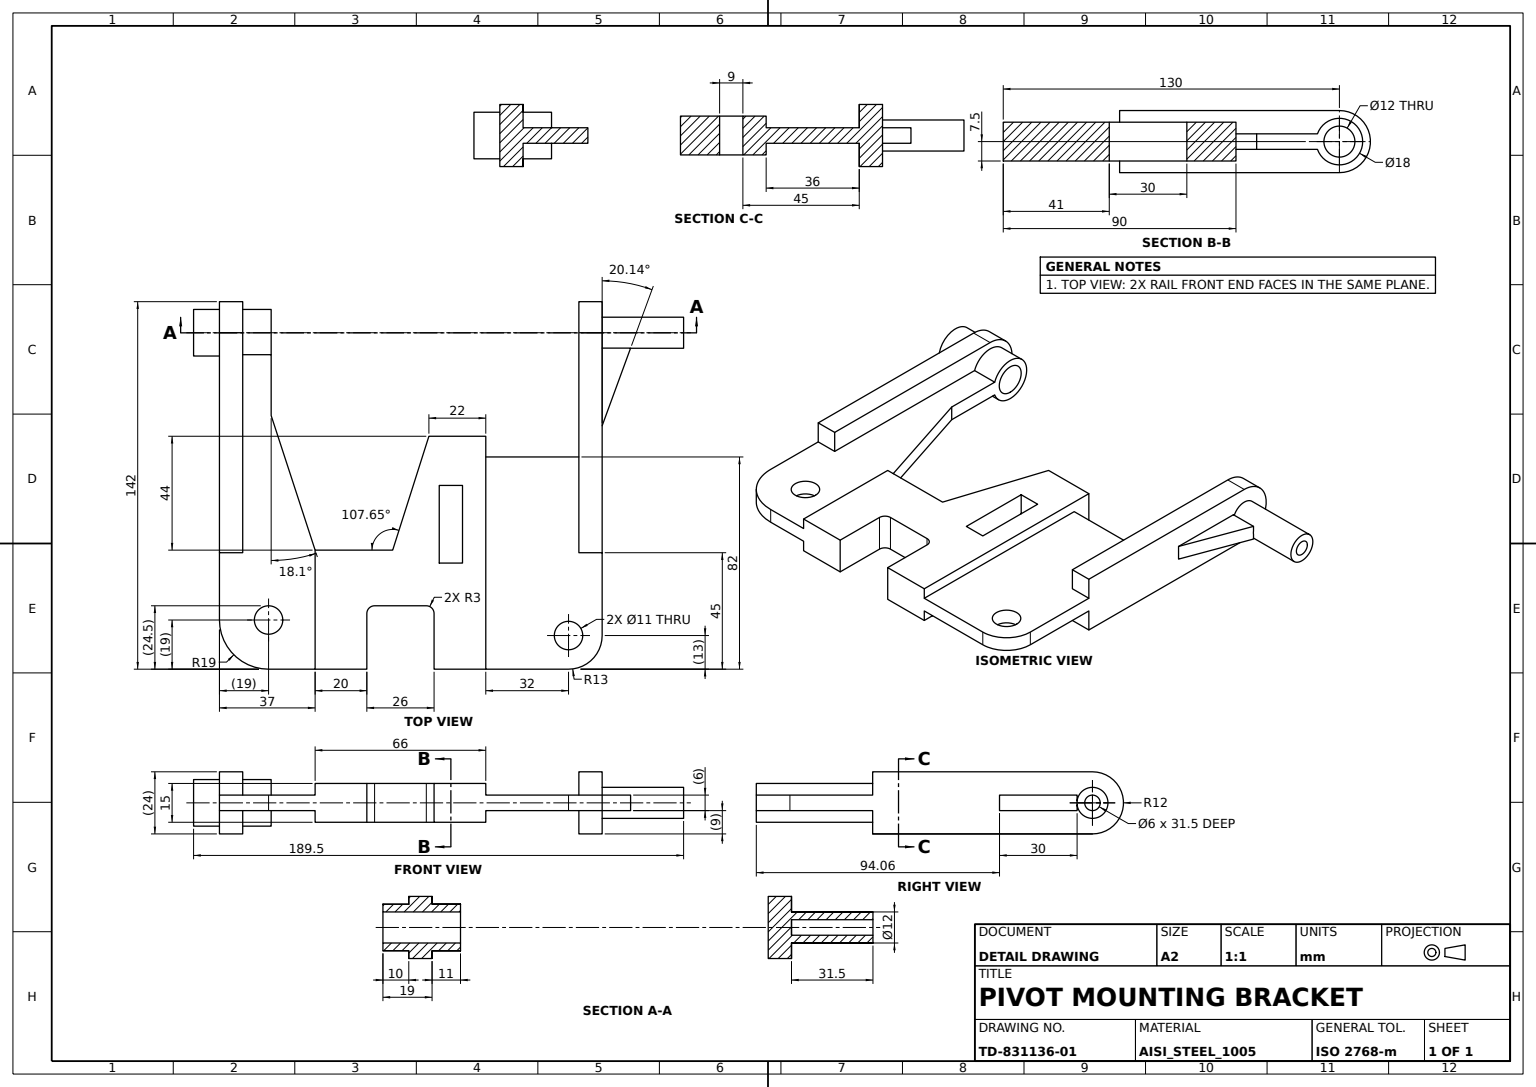
ISO-10303-21;
HEADER;
FILE_DESCRIPTION((''),'2;1');
FILE_NAME('','',(''),(''),'','','');
FILE_SCHEMA(('AUTOMOTIVE_DESIGN'));
ENDSEC;
DATA;
#1=APPLICATION_CONTEXT('');
#2=PRODUCT_CONTEXT('',#1,'mechanical');
#3=PRODUCT('','','',(#2));
#4=PRODUCT_DEFINITION_FORMATION('','',#3);
#5=PRODUCT_DEFINITION_CONTEXT('',#1,'design');
#6=PRODUCT_DEFINITION('','',#4,#5);
#7=PRODUCT_DEFINITION_SHAPE('','',#6);
#8=(LENGTH_UNIT()NAMED_UNIT(*)SI_UNIT(.MILLI.,.METRE.));
#9=(NAMED_UNIT(*)PLANE_ANGLE_UNIT()SI_UNIT($,.RADIAN.));
#10=(NAMED_UNIT(*)SI_UNIT($,.STERADIAN.)SOLID_ANGLE_UNIT());
#11=UNCERTAINTY_MEASURE_WITH_UNIT(LENGTH_MEASURE(0.005),#8,'distance_accuracy_value','');
#12=(GEOMETRIC_REPRESENTATION_CONTEXT(3)GLOBAL_UNCERTAINTY_ASSIGNED_CONTEXT((#11))GLOBAL_UNIT_ASSIGNED_CONTEXT((#8,#9,#10))REPRESENTATION_CONTEXT('',''));
#13=CARTESIAN_POINT('',(-80.,121.,0.));
#14=VERTEX_POINT('',#13);
#15=CARTESIAN_POINT('',(-80.,130.,0.));
#16=DIRECTION('',(-1.,0.,0.));
#17=DIRECTION('',(0.,-1.,0.));
#18=AXIS2_PLACEMENT_3D('',#15,#16,#17);
#19=CIRCLE('',#18,9.);
#20=EDGE_CURVE('',#14,#14,#19,.T.);
#21=ORIENTED_EDGE('',*,*,#20,.T.);
#22=EDGE_LOOP('',(#21));
#23=FACE_BOUND('',#22,.T.);
#24=CARTESIAN_POINT('',(-80.,130.,6.));
#25=VERTEX_POINT('',#24);
#26=DIRECTION('',(0.,0.,1.));
#27=AXIS2_PLACEMENT_3D('',#15,#16,#26);
#28=CIRCLE('',#27,6.);
#29=EDGE_CURVE('',#25,#25,#28,.F.);
#30=ORIENTED_EDGE('',*,*,#29,.T.);
#31=EDGE_LOOP('',(#30));
#32=FACE_BOUND('',#31,.T.);
#33=PLANE('',#27);
#34=ADVANCED_FACE('',(#23,#32),#33,.T.);
#35=CARTESIAN_POINT('',(78.,124.056727,-0.823106));
#36=VERTEX_POINT('',#35);
#37=CARTESIAN_POINT('',(89.,124.056727,-0.823106));
#38=VERTEX_POINT('',#37);
#39=CARTESIAN_POINT('',(109.5,124.056727,-0.823106));
#40=VECTOR('',#16,1000.);
#41=LINE('',#39,#40);
#42=EDGE_CURVE('',#36,#38,#41,.F.);
#43=ORIENTED_EDGE('',*,*,#42,.T.);
#44=CARTESIAN_POINT('',(89.,124.056727,-3.));
#45=VERTEX_POINT('',#44);
#46=CARTESIAN_POINT('',(89.,124.056727,3.));
#47=DIRECTION('',(0.,0.,-1.));
#48=VECTOR('',#47,1000.);
#49=LINE('',#46,#48);
#50=EDGE_CURVE('',#38,#45,#49,.T.);
#51=ORIENTED_EDGE('',*,*,#50,.T.);
#52=CARTESIAN_POINT('',(78.,124.056727,-3.));
#53=VERTEX_POINT('',#52);
#54=LINE('',#44,#40);
#55=EDGE_CURVE('',#45,#53,#54,.T.);
#56=ORIENTED_EDGE('',*,*,#55,.T.);
#57=CARTESIAN_POINT('',(78.,124.056727,3.));
#58=LINE('',#57,#48);
#59=EDGE_CURVE('',#36,#53,#58,.T.);
#60=ORIENTED_EDGE('',*,*,#59,.F.);
#61=EDGE_LOOP('',(#43,#51,#56,#60));
#62=FACE_BOUND('',#61,.T.);
#63=AXIS2_PLACEMENT_3D('',#46,#17,#47);
#64=PLANE('',#63);
#65=ADVANCED_FACE('',(#62),#64,.F.);
#66=CARTESIAN_POINT('',(-13.,21.5,-7.5));
#67=VERTEX_POINT('',#66);
#68=CARTESIAN_POINT('',(-13.,0.,-7.5));
#69=VERTEX_POINT('',#68);
#70=VECTOR('',#17,1000.);
#71=LINE('',#66,#70);
#72=EDGE_CURVE('',#67,#69,#71,.T.);
#73=ORIENTED_EDGE('',*,*,#72,.F.);
#74=CARTESIAN_POINT('',(-13.,21.5,7.5));
#75=VERTEX_POINT('',#74);
#76=LINE('',#74,#48);
#77=EDGE_CURVE('',#75,#67,#76,.T.);
#78=ORIENTED_EDGE('',*,*,#77,.F.);
#79=CARTESIAN_POINT('',(-13.,0.,7.5));
#80=VERTEX_POINT('',#79);
#81=LINE('',#74,#70);
#82=EDGE_CURVE('',#75,#80,#81,.T.);
#83=ORIENTED_EDGE('',*,*,#82,.T.);
#84=LINE('',#79,#48);
#85=EDGE_CURVE('',#80,#69,#84,.T.);
#86=ORIENTED_EDGE('',*,*,#85,.T.);
#87=EDGE_LOOP('',(#73,#78,#83,#86));
#88=FACE_BOUND('',#87,.T.);
#89=DIRECTION('',(1.,0.,0.));
#90=DIRECTION('',(0.,1.,0.));
#91=AXIS2_PLACEMENT_3D('',#74,#89,#90);
#92=PLANE('',#91);
#93=ADVANCED_FACE('',(#88),#92,.T.);
#94=CARTESIAN_POINT('',(-50.,98.,3.));
#95=VERTEX_POINT('',#94);
#96=CARTESIAN_POINT('',(-50.,98.,-3.));
#97=VERTEX_POINT('',#96);
#98=LINE('',#94,#48);
#99=EDGE_CURVE('',#95,#97,#98,.T.);
#100=ORIENTED_EDGE('',*,*,#99,.F.);
#101=CARTESIAN_POINT('',(-33.,46.,3.));
#102=VERTEX_POINT('',#101);
#103=DIRECTION('',(0.310738856,-0.950495325,0.));
#104=VECTOR('',#103,1000.);
#105=LINE('',#94,#104);
#106=EDGE_CURVE('',#95,#102,#105,.T.);
#107=ORIENTED_EDGE('',*,*,#106,.T.);
#108=CARTESIAN_POINT('',(-33.,46.,-3.));
#109=VERTEX_POINT('',#108);
#110=LINE('',#101,#48);
#111=EDGE_CURVE('',#102,#109,#110,.T.);
#112=ORIENTED_EDGE('',*,*,#111,.T.);
#113=LINE('',#96,#104);
#114=EDGE_CURVE('',#97,#109,#113,.T.);
#115=ORIENTED_EDGE('',*,*,#114,.F.);
#116=EDGE_LOOP('',(#100,#107,#112,#115));
#117=FACE_BOUND('',#116,.T.);
#118=DIRECTION('',(0.950495325,0.310738856,0.));
#119=DIRECTION('',(-0.310738856,0.950495325,0.));
#120=AXIS2_PLACEMENT_3D('',#94,#118,#119);
#121=PLANE('',#120);
#122=ADVANCED_FACE('',(#117),#121,.T.);
#123=CARTESIAN_POINT('',(69.,45.,-12.));
#124=VERTEX_POINT('',#123);
#125=CARTESIAN_POINT('',(69.,130.,-12.));
#126=VERTEX_POINT('',#125);
#127=VECTOR('',#90,1000.);
#128=LINE('',#123,#127);
#129=EDGE_CURVE('',#124,#126,#128,.T.);
#130=ORIENTED_EDGE('',*,*,#129,.T.);
#131=CARTESIAN_POINT('',(78.,130.,-12.));
#132=VERTEX_POINT('',#131);
#133=LINE('',#131,#40);
#134=EDGE_CURVE('',#132,#126,#133,.T.);
#135=ORIENTED_EDGE('',*,*,#134,.F.);
#136=CARTESIAN_POINT('',(78.,45.,-12.));
#137=VERTEX_POINT('',#136);
#138=LINE('',#136,#127);
#139=EDGE_CURVE('',#137,#132,#138,.T.);
#140=ORIENTED_EDGE('',*,*,#139,.F.);
#141=LINE('',#136,#40);
#142=EDGE_CURVE('',#137,#124,#141,.T.);
#143=ORIENTED_EDGE('',*,*,#142,.T.);
#144=EDGE_LOOP('',(#130,#135,#140,#143));
#145=FACE_BOUND('',#144,.T.);
#146=AXIS2_PLACEMENT_3D('',#136,#26,#17);
#147=PLANE('',#146);
#148=ADVANCED_FACE('',(#145),#147,.F.);
#149=CARTESIAN_POINT('',(-33.,0.,3.));
#150=VERTEX_POINT('',#149);
#151=CARTESIAN_POINT('',(-51.,0.,3.));
#152=VERTEX_POINT('',#151);
#153=LINE('',#149,#40);
#154=EDGE_CURVE('',#150,#152,#153,.T.);
#155=ORIENTED_EDGE('',*,*,#154,.T.);
#156=CARTESIAN_POINT('',(-51.,0.,-3.));
#157=VERTEX_POINT('',#156);
#158=LINE('',#151,#48);
#159=EDGE_CURVE('',#152,#157,#158,.T.);
#160=ORIENTED_EDGE('',*,*,#159,.T.);
#161=CARTESIAN_POINT('',(-33.,0.,-3.));
#162=VERTEX_POINT('',#161);
#163=LINE('',#161,#40);
#164=EDGE_CURVE('',#162,#157,#163,.T.);
#165=ORIENTED_EDGE('',*,*,#164,.F.);
#166=CARTESIAN_POINT('',(-33.,0.,-7.5));
#167=VERTEX_POINT('',#166);
#168=CARTESIAN_POINT('',(-33.,0.,7.5));
#169=LINE('',#168,#48);
#170=EDGE_CURVE('',#162,#167,#169,.T.);
#171=ORIENTED_EDGE('',*,*,#170,.T.);
#172=LINE('',#68,#40);
#173=EDGE_CURVE('',#69,#167,#172,.T.);
#174=ORIENTED_EDGE('',*,*,#173,.F.);
#175=ORIENTED_EDGE('',*,*,#85,.F.);
#176=VERTEX_POINT('',#168);
#177=LINE('',#79,#40);
#178=EDGE_CURVE('',#80,#176,#177,.T.);
#179=ORIENTED_EDGE('',*,*,#178,.T.);
#180=EDGE_CURVE('',#176,#150,#169,.T.);
#181=ORIENTED_EDGE('',*,*,#180,.T.);
#182=EDGE_LOOP('',(#155,#160,#165,#171,#174,#175,#179,#181));
#183=FACE_BOUND('',#182,.T.);
#184=AXIS2_PLACEMENT_3D('',#79,#17,#89);
#185=PLANE('',#184);
#186=ADVANCED_FACE('',(#183),#185,.T.);
#187=CARTESIAN_POINT('',(33.,0.,7.5));
#188=VERTEX_POINT('',#187);
#189=CARTESIAN_POINT('',(33.,0.,3.));
#190=VERTEX_POINT('',#189);
#191=LINE('',#187,#48);
#192=EDGE_CURVE('',#188,#190,#191,.T.);
#193=ORIENTED_EDGE('',*,*,#192,.F.);
#194=CARTESIAN_POINT('',(13.,0.,7.5));
#195=VERTEX_POINT('',#194);
#196=LINE('',#187,#40);
#197=EDGE_CURVE('',#188,#195,#196,.T.);
#198=ORIENTED_EDGE('',*,*,#197,.T.);
#199=CARTESIAN_POINT('',(13.,0.,-7.5));
#200=VERTEX_POINT('',#199);
#201=LINE('',#194,#48);
#202=EDGE_CURVE('',#195,#200,#201,.T.);
#203=ORIENTED_EDGE('',*,*,#202,.T.);
#204=CARTESIAN_POINT('',(33.,0.,-7.5));
#205=VERTEX_POINT('',#204);
#206=LINE('',#204,#40);
#207=EDGE_CURVE('',#205,#200,#206,.T.);
#208=ORIENTED_EDGE('',*,*,#207,.F.);
#209=CARTESIAN_POINT('',(33.,0.,-3.));
#210=VERTEX_POINT('',#209);
#211=EDGE_CURVE('',#210,#205,#191,.T.);
#212=ORIENTED_EDGE('',*,*,#211,.F.);
#213=CARTESIAN_POINT('',(65.,0.,-3.));
#214=VERTEX_POINT('',#213);
#215=LINE('',#213,#40);
#216=EDGE_CURVE('',#214,#210,#215,.T.);
#217=ORIENTED_EDGE('',*,*,#216,.F.);
#218=CARTESIAN_POINT('',(65.,0.,3.));
#219=VERTEX_POINT('',#218);
#220=LINE('',#218,#48);
#221=EDGE_CURVE('',#219,#214,#220,.T.);
#222=ORIENTED_EDGE('',*,*,#221,.F.);
#223=LINE('',#218,#40);
#224=EDGE_CURVE('',#219,#190,#223,.T.);
#225=ORIENTED_EDGE('',*,*,#224,.T.);
#226=EDGE_LOOP('',(#193,#198,#203,#208,#212,#217,#222,#225));
#227=FACE_BOUND('',#226,.T.);
#228=AXIS2_PLACEMENT_3D('',#187,#17,#89);
#229=PLANE('',#228);
#230=ADVANCED_FACE('',(#227),#229,.T.);
#231=CARTESIAN_POINT('',(78.,94.056727,3.));
#232=VERTEX_POINT('',#231);
#233=VERTEX_POINT('',#46);
#234=DIRECTION('',(0.344254649,0.938876316,0.));
#235=VECTOR('',#234,1000.);
#236=LINE('',#231,#235);
#237=EDGE_CURVE('',#232,#233,#236,.T.);
#238=ORIENTED_EDGE('',*,*,#237,.T.);
#239=VERTEX_POINT('',#57);
#240=LINE('',#46,#40);
#241=EDGE_CURVE('',#233,#239,#240,.T.);
#242=ORIENTED_EDGE('',*,*,#241,.T.);
#243=LINE('',#57,#70);
#244=EDGE_CURVE('',#239,#232,#243,.T.);
#245=ORIENTED_EDGE('',*,*,#244,.T.);
#246=EDGE_LOOP('',(#238,#242,#245));
#247=FACE_BOUND('',#246,.T.);
#248=CARTESIAN_POINT('',(0.,0.,3.));
#249=AXIS2_PLACEMENT_3D('',#248,#47,#16);
#250=PLANE('',#249);
#251=ADVANCED_FACE('',(#247),#250,.F.);
#252=CARTESIAN_POINT('',(69.,45.,-3.));
#253=VERTEX_POINT('',#252);
#254=CARTESIAN_POINT('',(69.,45.,12.));
#255=LINE('',#254,#48);
#256=EDGE_CURVE('',#253,#124,#255,.T.);
#257=ORIENTED_EDGE('',*,*,#256,.T.);
#258=ORIENTED_EDGE('',*,*,#142,.F.);
#259=CARTESIAN_POINT('',(78.,45.,-3.));
#260=VERTEX_POINT('',#259);
#261=CARTESIAN_POINT('',(78.,45.,12.));
#262=LINE('',#261,#48);
#263=EDGE_CURVE('',#260,#137,#262,.T.);
#264=ORIENTED_EDGE('',*,*,#263,.F.);
#265=VECTOR('',#89,1000.);
#266=LINE('',#252,#265);
#267=EDGE_CURVE('',#253,#260,#266,.T.);
#268=ORIENTED_EDGE('',*,*,#267,.F.);
#269=EDGE_LOOP('',(#257,#258,#264,#268));
#270=FACE_BOUND('',#269,.T.);
#271=AXIS2_PLACEMENT_3D('',#261,#90,#26);
#272=PLANE('',#271);
#273=ADVANCED_FACE('',(#270),#272,.F.);
#274=CARTESIAN_POINT('',(-3.,46.,-7.5));
#275=VERTEX_POINT('',#274);
#276=CARTESIAN_POINT('',(11.,90.,-7.5));
#277=VERTEX_POINT('',#276);
#278=DIRECTION('',(0.303203657,0.95292578,0.));
#279=VECTOR('',#278,1000.);
#280=LINE('',#274,#279);
#281=EDGE_CURVE('',#275,#277,#280,.T.);
#282=ORIENTED_EDGE('',*,*,#281,.F.);
#283=CARTESIAN_POINT('',(-3.,46.,7.5));
#284=VERTEX_POINT('',#283);
#285=LINE('',#283,#48);
#286=EDGE_CURVE('',#284,#275,#285,.T.);
#287=ORIENTED_EDGE('',*,*,#286,.F.);
#288=CARTESIAN_POINT('',(11.,90.,7.5));
#289=VERTEX_POINT('',#288);
#290=LINE('',#283,#279);
#291=EDGE_CURVE('',#284,#289,#290,.T.);
#292=ORIENTED_EDGE('',*,*,#291,.T.);
#293=LINE('',#288,#48);
#294=EDGE_CURVE('',#289,#277,#293,.T.);
#295=ORIENTED_EDGE('',*,*,#294,.T.);
#296=EDGE_LOOP('',(#282,#287,#292,#295));
#297=FACE_BOUND('',#296,.T.);
#298=DIRECTION('',(-0.95292578,0.303203657,0.));
#299=DIRECTION('',(-0.303203657,-0.95292578,0.));
#300=AXIS2_PLACEMENT_3D('',#283,#298,#299);
#301=PLANE('',#300);
#302=ADVANCED_FACE('',(#297),#301,.T.);
#303=CARTESIAN_POINT('',(-61.,45.,12.));
#304=VERTEX_POINT('',#303);
#305=CARTESIAN_POINT('',(-61.,45.,3.));
#306=VERTEX_POINT('',#305);
#307=LINE('',#303,#48);
#308=EDGE_CURVE('',#304,#306,#307,.T.);
#309=ORIENTED_EDGE('',*,*,#308,.F.);
#310=CARTESIAN_POINT('',(-70.,45.,12.));
#311=VERTEX_POINT('',#310);
#312=LINE('',#310,#265);
#313=EDGE_CURVE('',#311,#304,#312,.T.);
#314=ORIENTED_EDGE('',*,*,#313,.F.);
#315=CARTESIAN_POINT('',(-70.,45.,3.));
#316=VERTEX_POINT('',#315);
#317=LINE('',#310,#48);
#318=EDGE_CURVE('',#311,#316,#317,.T.);
#319=ORIENTED_EDGE('',*,*,#318,.T.);
#320=LINE('',#315,#265);
#321=EDGE_CURVE('',#316,#306,#320,.T.);
#322=ORIENTED_EDGE('',*,*,#321,.T.);
#323=EDGE_LOOP('',(#309,#314,#319,#322));
#324=FACE_BOUND('',#323,.T.);
#325=AXIS2_PLACEMENT_3D('',#310,#17,#89);
#326=PLANE('',#325);
#327=ADVANCED_FACE('',(#324),#326,.T.);
#328=CARTESIAN_POINT('',(78.,130.,12.));
#329=VERTEX_POINT('',#328);
#330=CARTESIAN_POINT('',(69.,130.,12.));
#331=VERTEX_POINT('',#330);
#332=LINE('',#328,#40);
#333=EDGE_CURVE('',#329,#331,#332,.T.);
#334=ORIENTED_EDGE('',*,*,#333,.T.);
#335=VERTEX_POINT('',#254);
#336=LINE('',#330,#70);
#337=EDGE_CURVE('',#331,#335,#336,.T.);
#338=ORIENTED_EDGE('',*,*,#337,.T.);
#339=VERTEX_POINT('',#261);
#340=LINE('',#261,#40);
#341=EDGE_CURVE('',#339,#335,#340,.T.);
#342=ORIENTED_EDGE('',*,*,#341,.F.);
#343=LINE('',#328,#70);
#344=EDGE_CURVE('',#329,#339,#343,.T.);
#345=ORIENTED_EDGE('',*,*,#344,.F.);
#346=EDGE_LOOP('',(#334,#338,#342,#345));
#347=FACE_BOUND('',#346,.T.);
#348=AXIS2_PLACEMENT_3D('',#328,#47,#90);
#349=PLANE('',#348);
#350=ADVANCED_FACE('',(#347),#349,.F.);
#351=CARTESIAN_POINT('',(78.,130.,-3.));
#352=VERTEX_POINT('',#351);
#353=CARTESIAN_POINT('',(78.,130.,0.));
#354=AXIS2_PLACEMENT_3D('',#353,#89,#47);
#355=CIRCLE('',#354,3.);
#356=EDGE_CURVE('',#352,#352,#355,.F.);
#357=ORIENTED_EDGE('',*,*,#356,.F.);
#358=EDGE_LOOP('',(#357));
#359=FACE_BOUND('',#358,.T.);
#360=CARTESIAN_POINT('',(78.,45.,3.));
#361=AXIS2_PLACEMENT_3D('',#360,#89,#47);
#362=PLANE('',#361);
#363=ADVANCED_FACE('',(#359),#362,.T.);
#364=CARTESIAN_POINT('',(24.,41.,-7.5));
#365=VERTEX_POINT('',#364);
#366=CARTESIAN_POINT('',(15.,41.,-7.5));
#367=VERTEX_POINT('',#366);
#368=LINE('',#364,#40);
#369=EDGE_CURVE('',#365,#367,#368,.T.);
#370=ORIENTED_EDGE('',*,*,#369,.T.);
#371=CARTESIAN_POINT('',(15.,41.,7.5));
#372=VERTEX_POINT('',#371);
#373=LINE('',#371,#48);
#374=EDGE_CURVE('',#372,#367,#373,.T.);
#375=ORIENTED_EDGE('',*,*,#374,.F.);
#376=CARTESIAN_POINT('',(24.,41.,7.5));
#377=VERTEX_POINT('',#376);
#378=LINE('',#376,#40);
#379=EDGE_CURVE('',#377,#372,#378,.T.);
#380=ORIENTED_EDGE('',*,*,#379,.F.);
#381=LINE('',#376,#48);
#382=EDGE_CURVE('',#377,#365,#381,.T.);
#383=ORIENTED_EDGE('',*,*,#382,.T.);
#384=EDGE_LOOP('',(#370,#375,#380,#383));
#385=FACE_BOUND('',#384,.T.);
#386=AXIS2_PLACEMENT_3D('',#376,#17,#47);
#387=PLANE('',#386);
#388=ADVANCED_FACE('',(#385),#387,.F.);
#389=CARTESIAN_POINT('',(15.,71.,-7.5));
#390=VERTEX_POINT('',#389);
#391=CARTESIAN_POINT('',(24.,71.,-7.5));
#392=VERTEX_POINT('',#391);
#393=LINE('',#389,#265);
#394=EDGE_CURVE('',#390,#392,#393,.T.);
#395=ORIENTED_EDGE('',*,*,#394,.T.);
#396=CARTESIAN_POINT('',(24.,71.,7.5));
#397=VERTEX_POINT('',#396);
#398=LINE('',#396,#48);
#399=EDGE_CURVE('',#397,#392,#398,.T.);
#400=ORIENTED_EDGE('',*,*,#399,.F.);
#401=CARTESIAN_POINT('',(15.,71.,7.5));
#402=VERTEX_POINT('',#401);
#403=LINE('',#401,#265);
#404=EDGE_CURVE('',#402,#397,#403,.T.);
#405=ORIENTED_EDGE('',*,*,#404,.F.);
#406=LINE('',#401,#48);
#407=EDGE_CURVE('',#402,#390,#406,.T.);
#408=ORIENTED_EDGE('',*,*,#407,.T.);
#409=EDGE_LOOP('',(#395,#400,#405,#408));
#410=FACE_BOUND('',#409,.T.);
#411=AXIS2_PLACEMENT_3D('',#401,#90,#26);
#412=PLANE('',#411);
#413=ADVANCED_FACE('',(#410),#412,.F.);
#414=CARTESIAN_POINT('',(-70.,45.,-12.));
#415=VERTEX_POINT('',#414);
#416=CARTESIAN_POINT('',(-61.,45.,-12.));
#417=VERTEX_POINT('',#416);
#418=LINE('',#414,#265);
#419=EDGE_CURVE('',#415,#417,#418,.T.);
#420=ORIENTED_EDGE('',*,*,#419,.T.);
#421=CARTESIAN_POINT('',(-61.,45.,-3.));
#422=VERTEX_POINT('',#421);
#423=EDGE_CURVE('',#422,#417,#307,.T.);
#424=ORIENTED_EDGE('',*,*,#423,.F.);
#425=CARTESIAN_POINT('',(-70.,45.,-3.));
#426=VERTEX_POINT('',#425);
#427=LINE('',#425,#265);
#428=EDGE_CURVE('',#426,#422,#427,.T.);
#429=ORIENTED_EDGE('',*,*,#428,.F.);
#430=EDGE_CURVE('',#426,#415,#317,.T.);
#431=ORIENTED_EDGE('',*,*,#430,.T.);
#432=EDGE_LOOP('',(#420,#424,#429,#431));
#433=FACE_BOUND('',#432,.T.);
#434=ADVANCED_FACE('',(#433),#326,.T.);
#435=CARTESIAN_POINT('',(33.,82.,-3.));
#436=VERTEX_POINT('',#435);
#437=LINE('',#209,#127);
#438=EDGE_CURVE('',#210,#436,#437,.T.);
#439=ORIENTED_EDGE('',*,*,#438,.F.);
#440=ORIENTED_EDGE('',*,*,#211,.T.);
#441=CARTESIAN_POINT('',(33.,90.,-7.5));
#442=VERTEX_POINT('',#441);
#443=LINE('',#441,#70);
#444=EDGE_CURVE('',#442,#205,#443,.T.);
#445=ORIENTED_EDGE('',*,*,#444,.F.);
#446=CARTESIAN_POINT('',(33.,90.,7.5));
#447=VERTEX_POINT('',#446);
#448=LINE('',#446,#48);
#449=EDGE_CURVE('',#447,#442,#448,.T.);
#450=ORIENTED_EDGE('',*,*,#449,.F.);
#451=LINE('',#446,#70);
#452=EDGE_CURVE('',#447,#188,#451,.T.);
#453=ORIENTED_EDGE('',*,*,#452,.T.);
#454=ORIENTED_EDGE('',*,*,#192,.T.);
#455=CARTESIAN_POINT('',(33.,82.,3.));
#456=VERTEX_POINT('',#455);
#457=LINE('',#189,#127);
#458=EDGE_CURVE('',#190,#456,#457,.T.);
#459=ORIENTED_EDGE('',*,*,#458,.T.);
#460=LINE('',#455,#48);
#461=EDGE_CURVE('',#456,#436,#460,.T.);
#462=ORIENTED_EDGE('',*,*,#461,.T.);
#463=EDGE_LOOP('',(#439,#440,#445,#450,#453,#454,#459,#462));
#464=FACE_BOUND('',#463,.T.);
#465=AXIS2_PLACEMENT_3D('',#446,#89,#47);
#466=PLANE('',#465);
#467=ADVANCED_FACE('',(#464),#466,.T.);
#468=CARTESIAN_POINT('',(-50.,121.514719,-3.));
#469=VERTEX_POINT('',#468);
#470=CARTESIAN_POINT('',(-50.,121.514719,3.));
#471=VERTEX_POINT('',#470);
#472=CARTESIAN_POINT('',(-50.,130.,0.));
#473=AXIS2_PLACEMENT_3D('',#472,#89,#90);
#474=CIRCLE('',#473,9.);
#475=EDGE_CURVE('',#469,#471,#474,.T.);
#476=ORIENTED_EDGE('',*,*,#475,.T.);
#477=CARTESIAN_POINT('',(-50.,130.,3.));
#478=LINE('',#477,#70);
#479=EDGE_CURVE('',#471,#95,#478,.T.);
#480=ORIENTED_EDGE('',*,*,#479,.T.);
#481=ORIENTED_EDGE('',*,*,#99,.T.);
#482=CARTESIAN_POINT('',(-50.,130.,-3.));
#483=LINE('',#482,#70);
#484=EDGE_CURVE('',#469,#97,#483,.T.);
#485=ORIENTED_EDGE('',*,*,#484,.F.);
#486=EDGE_LOOP('',(#476,#480,#481,#485));
#487=FACE_BOUND('',#486,.T.);
#488=CARTESIAN_POINT('',(-50.,130.,-6.));
#489=VERTEX_POINT('',#488);
#490=AXIS2_PLACEMENT_3D('',#472,#89,#47);
#491=CIRCLE('',#490,6.);
#492=EDGE_CURVE('',#489,#489,#491,.F.);
#493=ORIENTED_EDGE('',*,*,#492,.T.);
#494=EDGE_LOOP('',(#493));
#495=FACE_BOUND('',#494,.T.);
#496=AXIS2_PLACEMENT_3D('',#477,#89,#47);
#497=PLANE('',#496);
#498=ADVANCED_FACE('',(#487,#495),#497,.T.);
#499=CARTESIAN_POINT('',(-70.,19.,3.));
#500=VERTEX_POINT('',#499);
#501=CARTESIAN_POINT('',(-70.,19.,-3.));
#502=VERTEX_POINT('',#501);
#503=LINE('',#499,#48);
#504=EDGE_CURVE('',#500,#502,#503,.T.);
#505=ORIENTED_EDGE('',*,*,#504,.T.);
#506=CARTESIAN_POINT('',(-51.,19.,-3.));
#507=AXIS2_PLACEMENT_3D('',#506,#47,#89);
#508=CIRCLE('',#507,19.);
#509=EDGE_CURVE('',#157,#502,#508,.T.);
#510=ORIENTED_EDGE('',*,*,#509,.F.);
#511=ORIENTED_EDGE('',*,*,#159,.F.);
#512=CARTESIAN_POINT('',(-51.,19.,3.));
#513=AXIS2_PLACEMENT_3D('',#512,#47,#89);
#514=CIRCLE('',#513,19.);
#515=EDGE_CURVE('',#152,#500,#514,.T.);
#516=ORIENTED_EDGE('',*,*,#515,.T.);
#517=EDGE_LOOP('',(#505,#510,#511,#516));
#518=FACE_BOUND('',#517,.T.);
#519=AXIS2_PLACEMENT_3D('',#512,#47,#16);
#520=CYLINDRICAL_SURFACE('',#519,19.);
#521=ADVANCED_FACE('',(#518),#520,.T.);
#522=ORIENTED_EDGE('',*,*,#407,.F.);
#523=LINE('',#371,#127);
#524=EDGE_CURVE('',#372,#402,#523,.T.);
#525=ORIENTED_EDGE('',*,*,#524,.F.);
#526=ORIENTED_EDGE('',*,*,#374,.T.);
#527=LINE('',#366,#127);
#528=EDGE_CURVE('',#367,#390,#527,.T.);
#529=ORIENTED_EDGE('',*,*,#528,.T.);
#530=EDGE_LOOP('',(#522,#525,#526,#529));
#531=FACE_BOUND('',#530,.T.);
#532=AXIS2_PLACEMENT_3D('',#371,#16,#17);
#533=PLANE('',#532);
#534=ADVANCED_FACE('',(#531),#533,.F.);
#535=CARTESIAN_POINT('',(-33.,46.,7.5));
#536=VERTEX_POINT('',#535);
#537=LINE('',#535,#48);
#538=EDGE_CURVE('',#536,#102,#537,.T.);
#539=ORIENTED_EDGE('',*,*,#538,.T.);
#540=LINE('',#101,#70);
#541=EDGE_CURVE('',#102,#150,#540,.T.);
#542=ORIENTED_EDGE('',*,*,#541,.T.);
#543=ORIENTED_EDGE('',*,*,#180,.F.);
#544=LINE('',#168,#127);
#545=EDGE_CURVE('',#176,#536,#544,.T.);
#546=ORIENTED_EDGE('',*,*,#545,.T.);
#547=EDGE_LOOP('',(#539,#542,#543,#546));
#548=FACE_BOUND('',#547,.T.);
#549=AXIS2_PLACEMENT_3D('',#168,#16,#26);
#550=PLANE('',#549);
#551=ADVANCED_FACE('',(#548),#550,.T.);
#552=CARTESIAN_POINT('',(-45.5,19.,-3.));
#553=VERTEX_POINT('',#552);
#554=AXIS2_PLACEMENT_3D('',#506,#26,#89);
#555=CIRCLE('',#554,5.5);
#556=EDGE_CURVE('',#553,#553,#555,.T.);
#557=ORIENTED_EDGE('',*,*,#556,.F.);
#558=EDGE_LOOP('',(#557));
#559=FACE_BOUND('',#558,.T.);
#560=CARTESIAN_POINT('',(-45.5,19.,3.));
#561=VERTEX_POINT('',#560);
#562=AXIS2_PLACEMENT_3D('',#512,#26,#89);
#563=CIRCLE('',#562,5.5);
#564=EDGE_CURVE('',#561,#561,#563,.T.);
#565=ORIENTED_EDGE('',*,*,#564,.T.);
#566=EDGE_LOOP('',(#565));
#567=FACE_BOUND('',#566,.T.);
#568=CYLINDRICAL_SURFACE('',#519,5.5);
#569=ADVANCED_FACE('',(#559,#567),#568,.F.);
#570=CARTESIAN_POINT('',(78.,94.056727,-3.));
#571=VERTEX_POINT('',#570);
#572=LINE('',#231,#48);
#573=EDGE_CURVE('',#232,#571,#572,.T.);
#574=ORIENTED_EDGE('',*,*,#573,.T.);
#575=LINE('',#570,#235);
#576=EDGE_CURVE('',#571,#45,#575,.T.);
#577=ORIENTED_EDGE('',*,*,#576,.T.);
#578=ORIENTED_EDGE('',*,*,#50,.F.);
#579=CARTESIAN_POINT('',(89.,124.056727,0.823106));
#580=VERTEX_POINT('',#579);
#581=CARTESIAN_POINT('',(91.1792,130.,0.));
#582=DIRECTION('',(-0.938876316,0.344254649,0.));
#583=DIRECTION('',(-0.344254649,-0.938876316,0.));
#584=AXIS2_PLACEMENT_3D('',#581,#582,#583);
#585=ELLIPSE('',#584,6.390618,6.);
#586=EDGE_CURVE('',#38,#580,#585,.T.);
#587=ORIENTED_EDGE('',*,*,#586,.T.);
#588=EDGE_CURVE('',#233,#580,#49,.T.);
#589=ORIENTED_EDGE('',*,*,#588,.F.);
#590=ORIENTED_EDGE('',*,*,#237,.F.);
#591=EDGE_LOOP('',(#574,#577,#578,#587,#589,#590));
#592=FACE_BOUND('',#591,.T.);
#593=AXIS2_PLACEMENT_3D('',#231,#582,#583);
#594=PLANE('',#593);
#595=ADVANCED_FACE('',(#592),#594,.F.);
#596=LINE('',#288,#265);
#597=EDGE_CURVE('',#289,#447,#596,.T.);
#598=ORIENTED_EDGE('',*,*,#597,.T.);
#599=ORIENTED_EDGE('',*,*,#449,.T.);
#600=LINE('',#276,#265);
#601=EDGE_CURVE('',#277,#442,#600,.T.);
#602=ORIENTED_EDGE('',*,*,#601,.F.);
#603=ORIENTED_EDGE('',*,*,#294,.F.);
#604=EDGE_LOOP('',(#598,#599,#602,#603));
#605=FACE_BOUND('',#604,.T.);
#606=AXIS2_PLACEMENT_3D('',#288,#90,#26);
#607=PLANE('',#606);
#608=ADVANCED_FACE('',(#605),#607,.T.);
#609=ORIENTED_EDGE('',*,*,#382,.F.);
#610=LINE('',#396,#70);
#611=EDGE_CURVE('',#397,#377,#610,.T.);
#612=ORIENTED_EDGE('',*,*,#611,.F.);
#613=ORIENTED_EDGE('',*,*,#399,.T.);
#614=LINE('',#391,#70);
#615=EDGE_CURVE('',#392,#365,#614,.T.);
#616=ORIENTED_EDGE('',*,*,#615,.T.);
#617=EDGE_LOOP('',(#609,#612,#613,#616));
#618=FACE_BOUND('',#617,.T.);
#619=AXIS2_PLACEMENT_3D('',#396,#89,#90);
#620=PLANE('',#619);
#621=ADVANCED_FACE('',(#618),#620,.F.);
#622=CARTESIAN_POINT('',(69.,82.,-3.));
#623=VERTEX_POINT('',#622);
#624=LINE('',#435,#265);
#625=EDGE_CURVE('',#436,#623,#624,.T.);
#626=ORIENTED_EDGE('',*,*,#625,.F.);
#627=ORIENTED_EDGE('',*,*,#461,.F.);
#628=CARTESIAN_POINT('',(69.,82.,3.));
#629=VERTEX_POINT('',#628);
#630=LINE('',#455,#265);
#631=EDGE_CURVE('',#456,#629,#630,.T.);
#632=ORIENTED_EDGE('',*,*,#631,.T.);
#633=LINE('',#628,#48);
#634=EDGE_CURVE('',#629,#623,#633,.T.);
#635=ORIENTED_EDGE('',*,*,#634,.T.);
#636=EDGE_LOOP('',(#626,#627,#632,#635));
#637=FACE_BOUND('',#636,.T.);
#638=AXIS2_PLACEMENT_3D('',#455,#90,#26);
#639=PLANE('',#638);
#640=ADVANCED_FACE('',(#637),#639,.T.);
#641=CARTESIAN_POINT('',(10.,24.5,-7.5));
#642=VERTEX_POINT('',#641);
#643=CARTESIAN_POINT('',(-10.,24.5,-7.5));
#644=VERTEX_POINT('',#643);
#645=LINE('',#641,#40);
#646=EDGE_CURVE('',#642,#644,#645,.T.);
#647=ORIENTED_EDGE('',*,*,#646,.T.);
#648=CARTESIAN_POINT('',(-10.,21.5,-7.5));
#649=AXIS2_PLACEMENT_3D('',#648,#26,#89);
#650=CIRCLE('',#649,3.);
#651=EDGE_CURVE('',#644,#67,#650,.T.);
#652=ORIENTED_EDGE('',*,*,#651,.T.);
#653=ORIENTED_EDGE('',*,*,#72,.T.);
#654=ORIENTED_EDGE('',*,*,#173,.T.);
#655=CARTESIAN_POINT('',(-33.,46.,-7.5));
#656=VERTEX_POINT('',#655);
#657=LINE('',#166,#127);
#658=EDGE_CURVE('',#167,#656,#657,.T.);
#659=ORIENTED_EDGE('',*,*,#658,.T.);
#660=LINE('',#655,#265);
#661=EDGE_CURVE('',#656,#275,#660,.T.);
#662=ORIENTED_EDGE('',*,*,#661,.T.);
#663=ORIENTED_EDGE('',*,*,#281,.T.);
#664=ORIENTED_EDGE('',*,*,#601,.T.);
#665=ORIENTED_EDGE('',*,*,#444,.T.);
#666=ORIENTED_EDGE('',*,*,#207,.T.);
#667=CARTESIAN_POINT('',(13.,21.5,-7.5));
#668=VERTEX_POINT('',#667);
#669=LINE('',#199,#127);
#670=EDGE_CURVE('',#200,#668,#669,.T.);
#671=ORIENTED_EDGE('',*,*,#670,.T.);
#672=CARTESIAN_POINT('',(10.,21.5,-7.5));
#673=AXIS2_PLACEMENT_3D('',#672,#26,#89);
#674=CIRCLE('',#673,3.);
#675=EDGE_CURVE('',#668,#642,#674,.T.);
#676=ORIENTED_EDGE('',*,*,#675,.T.);
#677=EDGE_LOOP('',(#647,#652,#653,#654,#659,#662,#663,#664,#665,#666,#671,#676));
#678=FACE_BOUND('',#677,.T.);
#679=ORIENTED_EDGE('',*,*,#369,.F.);
#680=ORIENTED_EDGE('',*,*,#615,.F.);
#681=ORIENTED_EDGE('',*,*,#394,.F.);
#682=ORIENTED_EDGE('',*,*,#528,.F.);
#683=EDGE_LOOP('',(#679,#680,#681,#682));
#684=FACE_BOUND('',#683,.T.);
#685=PLANE('',#673);
#686=ADVANCED_FACE('',(#678,#684),#685,.F.);
#687=CARTESIAN_POINT('',(109.5,133.,0.));
#688=VERTEX_POINT('',#687);
#689=CARTESIAN_POINT('',(109.5,130.,0.));
#690=AXIS2_PLACEMENT_3D('',#689,#89,#90);
#691=CIRCLE('',#690,3.);
#692=EDGE_CURVE('',#688,#688,#691,.T.);
#693=ORIENTED_EDGE('',*,*,#692,.T.);
#694=EDGE_LOOP('',(#693));
#695=FACE_BOUND('',#694,.T.);
#696=ORIENTED_EDGE('',*,*,#356,.T.);
#697=EDGE_LOOP('',(#696));
#698=FACE_BOUND('',#697,.T.);
#699=AXIS2_PLACEMENT_3D('',#689,#16,#26);
#700=CYLINDRICAL_SURFACE('',#699,3.);
#701=ADVANCED_FACE('',(#695,#698),#700,.F.);
#702=ORIENTED_EDGE('',*,*,#333,.F.);
#703=AXIS2_PLACEMENT_3D('',#353,#89,#90);
#704=CIRCLE('',#703,12.);
#705=EDGE_CURVE('',#132,#329,#704,.T.);
#706=ORIENTED_EDGE('',*,*,#705,.F.);
#707=ORIENTED_EDGE('',*,*,#134,.T.);
#708=CARTESIAN_POINT('',(69.,130.,0.));
#709=AXIS2_PLACEMENT_3D('',#708,#89,#90);
#710=CIRCLE('',#709,12.);
#711=EDGE_CURVE('',#126,#331,#710,.T.);
#712=ORIENTED_EDGE('',*,*,#711,.T.);
#713=EDGE_LOOP('',(#702,#706,#707,#712));
#714=FACE_BOUND('',#713,.T.);
#715=AXIS2_PLACEMENT_3D('',#353,#16,#26);
#716=CYLINDRICAL_SURFACE('',#715,12.);
#717=ADVANCED_FACE('',(#714),#716,.T.);
#718=CARTESIAN_POINT('',(78.,13.,3.));
#719=VERTEX_POINT('',#718);
#720=CARTESIAN_POINT('',(65.,13.,3.));
#721=AXIS2_PLACEMENT_3D('',#720,#47,#89);
#722=CIRCLE('',#721,13.);
#723=EDGE_CURVE('',#719,#219,#722,.T.);
#724=ORIENTED_EDGE('',*,*,#723,.T.);
#725=ORIENTED_EDGE('',*,*,#221,.T.);
#726=CARTESIAN_POINT('',(78.,13.,-3.));
#727=VERTEX_POINT('',#726);
#728=CARTESIAN_POINT('',(65.,13.,-3.));
#729=AXIS2_PLACEMENT_3D('',#728,#47,#89);
#730=CIRCLE('',#729,13.);
#731=EDGE_CURVE('',#727,#214,#730,.T.);
#732=ORIENTED_EDGE('',*,*,#731,.F.);
#733=LINE('',#718,#48);
#734=EDGE_CURVE('',#719,#727,#733,.T.);
#735=ORIENTED_EDGE('',*,*,#734,.F.);
#736=EDGE_LOOP('',(#724,#725,#732,#735));
#737=FACE_BOUND('',#736,.T.);
#738=AXIS2_PLACEMENT_3D('',#720,#47,#16);
#739=CYLINDRICAL_SURFACE('',#738,13.);
#740=ADVANCED_FACE('',(#737),#739,.T.);
#741=ORIENTED_EDGE('',*,*,#646,.F.);
#742=CARTESIAN_POINT('',(10.,24.5,7.5));
#743=VERTEX_POINT('',#742);
#744=LINE('',#742,#48);
#745=EDGE_CURVE('',#743,#642,#744,.T.);
#746=ORIENTED_EDGE('',*,*,#745,.F.);
#747=CARTESIAN_POINT('',(-10.,24.5,7.5));
#748=VERTEX_POINT('',#747);
#749=LINE('',#742,#40);
#750=EDGE_CURVE('',#743,#748,#749,.T.);
#751=ORIENTED_EDGE('',*,*,#750,.T.);
#752=LINE('',#747,#48);
#753=EDGE_CURVE('',#748,#644,#752,.T.);
#754=ORIENTED_EDGE('',*,*,#753,.T.);
#755=EDGE_LOOP('',(#741,#746,#751,#754));
#756=FACE_BOUND('',#755,.T.);
#757=AXIS2_PLACEMENT_3D('',#742,#17,#47);
#758=PLANE('',#757);
#759=ADVANCED_FACE('',(#756),#758,.T.);
#760=CARTESIAN_POINT('',(13.,21.5,7.5));
#761=VERTEX_POINT('',#760);
#762=LINE('',#194,#127);
#763=EDGE_CURVE('',#195,#761,#762,.T.);
#764=ORIENTED_EDGE('',*,*,#763,.T.);
#765=LINE('',#760,#48);
#766=EDGE_CURVE('',#761,#668,#765,.T.);
#767=ORIENTED_EDGE('',*,*,#766,.T.);
#768=ORIENTED_EDGE('',*,*,#670,.F.);
#769=ORIENTED_EDGE('',*,*,#202,.F.);
#770=EDGE_LOOP('',(#764,#767,#768,#769));
#771=FACE_BOUND('',#770,.T.);
#772=AXIS2_PLACEMENT_3D('',#194,#16,#17);
#773=PLANE('',#772);
#774=ADVANCED_FACE('',(#771),#773,.T.);
#775=CARTESIAN_POINT('',(-61.,121.514719,-3.));
#776=VERTEX_POINT('',#775);
#777=CARTESIAN_POINT('',(-61.,121.514719,3.));
#778=VERTEX_POINT('',#777);
#779=CARTESIAN_POINT('',(-61.,130.,0.));
#780=AXIS2_PLACEMENT_3D('',#779,#89,#90);
#781=CIRCLE('',#780,9.);
#782=EDGE_CURVE('',#776,#778,#781,.T.);
#783=ORIENTED_EDGE('',*,*,#782,.F.);
#784=LINE('',#421,#127);
#785=EDGE_CURVE('',#422,#776,#784,.T.);
#786=ORIENTED_EDGE('',*,*,#785,.F.);
#787=ORIENTED_EDGE('',*,*,#423,.T.);
#788=CARTESIAN_POINT('',(-61.,130.,-12.));
#789=VERTEX_POINT('',#788);
#790=LINE('',#416,#127);
#791=EDGE_CURVE('',#417,#789,#790,.T.);
#792=ORIENTED_EDGE('',*,*,#791,.T.);
#793=CARTESIAN_POINT('',(-61.,130.,12.));
#794=VERTEX_POINT('',#793);
#795=CIRCLE('',#780,12.);
#796=EDGE_CURVE('',#789,#794,#795,.T.);
#797=ORIENTED_EDGE('',*,*,#796,.T.);
#798=LINE('',#793,#70);
#799=EDGE_CURVE('',#794,#304,#798,.T.);
#800=ORIENTED_EDGE('',*,*,#799,.T.);
#801=ORIENTED_EDGE('',*,*,#308,.T.);
#802=LINE('',#305,#127);
#803=EDGE_CURVE('',#306,#778,#802,.T.);
#804=ORIENTED_EDGE('',*,*,#803,.T.);
#805=EDGE_LOOP('',(#783,#786,#787,#792,#797,#800,#801,#804));
#806=FACE_BOUND('',#805,.T.);
#807=AXIS2_PLACEMENT_3D('',#779,#89,#47);
#808=PLANE('',#807);
#809=ADVANCED_FACE('',(#806),#808,.T.);
#810=ORIENTED_EDGE('',*,*,#661,.F.);
#811=EDGE_CURVE('',#109,#656,#537,.T.);
#812=ORIENTED_EDGE('',*,*,#811,.F.);
#813=ORIENTED_EDGE('',*,*,#111,.F.);
#814=ORIENTED_EDGE('',*,*,#538,.F.);
#815=LINE('',#535,#265);
#816=EDGE_CURVE('',#536,#284,#815,.T.);
#817=ORIENTED_EDGE('',*,*,#816,.T.);
#818=ORIENTED_EDGE('',*,*,#286,.T.);
#819=EDGE_LOOP('',(#810,#812,#813,#814,#817,#818));
#820=FACE_BOUND('',#819,.T.);
#821=AXIS2_PLACEMENT_3D('',#535,#90,#26);
#822=PLANE('',#821);
#823=ADVANCED_FACE('',(#820),#822,.T.);
#824=CARTESIAN_POINT('',(-70.,130.,-12.));
#825=VERTEX_POINT('',#824);
#826=LINE('',#824,#265);
#827=EDGE_CURVE('',#825,#789,#826,.T.);
#828=ORIENTED_EDGE('',*,*,#827,.T.);
#829=ORIENTED_EDGE('',*,*,#791,.F.);
#830=ORIENTED_EDGE('',*,*,#419,.F.);
#831=LINE('',#414,#127);
#832=EDGE_CURVE('',#415,#825,#831,.T.);
#833=ORIENTED_EDGE('',*,*,#832,.T.);
#834=EDGE_LOOP('',(#828,#829,#830,#833));
#835=FACE_BOUND('',#834,.T.);
#836=AXIS2_PLACEMENT_3D('',#414,#47,#16);
#837=PLANE('',#836);
#838=ADVANCED_FACE('',(#835),#837,.T.);
#839=ORIENTED_EDGE('',*,*,#475,.F.);
#840=LINE('',#468,#40);
#841=EDGE_CURVE('',#776,#469,#840,.F.);
#842=ORIENTED_EDGE('',*,*,#841,.F.);
#843=ORIENTED_EDGE('',*,*,#782,.T.);
#844=LINE('',#470,#40);
#845=EDGE_CURVE('',#778,#471,#844,.F.);
#846=ORIENTED_EDGE('',*,*,#845,.T.);
#847=EDGE_LOOP('',(#839,#842,#843,#846));
#848=FACE_BOUND('',#847,.T.);
#849=AXIS2_PLACEMENT_3D('',#472,#16,#26);
#850=CYLINDRICAL_SURFACE('',#849,9.);
#851=ADVANCED_FACE('',(#848),#850,.T.);
#852=ORIENTED_EDGE('',*,*,#256,.F.);
#853=LINE('',#622,#70);
#854=EDGE_CURVE('',#623,#253,#853,.T.);
#855=ORIENTED_EDGE('',*,*,#854,.F.);
#856=ORIENTED_EDGE('',*,*,#634,.F.);
#857=CARTESIAN_POINT('',(69.,45.,3.));
#858=VERTEX_POINT('',#857);
#859=LINE('',#628,#70);
#860=EDGE_CURVE('',#629,#858,#859,.T.);
#861=ORIENTED_EDGE('',*,*,#860,.T.);
#862=EDGE_CURVE('',#335,#858,#255,.T.);
#863=ORIENTED_EDGE('',*,*,#862,.F.);
#864=ORIENTED_EDGE('',*,*,#337,.F.);
#865=ORIENTED_EDGE('',*,*,#711,.F.);
#866=ORIENTED_EDGE('',*,*,#129,.F.);
#867=EDGE_LOOP('',(#852,#855,#856,#861,#863,#864,#865,#866));
#868=FACE_BOUND('',#867,.T.);
#869=AXIS2_PLACEMENT_3D('',#708,#89,#47);
#870=PLANE('',#869);
#871=ADVANCED_FACE('',(#868),#870,.F.);
#872=CARTESIAN_POINT('',(-70.,130.,12.));
#873=VERTEX_POINT('',#872);
#874=LINE('',#872,#265);
#875=EDGE_CURVE('',#873,#794,#874,.T.);
#876=ORIENTED_EDGE('',*,*,#875,.T.);
#877=ORIENTED_EDGE('',*,*,#796,.F.);
#878=ORIENTED_EDGE('',*,*,#827,.F.);
#879=CARTESIAN_POINT('',(-70.,130.,0.));
#880=AXIS2_PLACEMENT_3D('',#879,#89,#90);
#881=CIRCLE('',#880,12.);
#882=EDGE_CURVE('',#825,#873,#881,.T.);
#883=ORIENTED_EDGE('',*,*,#882,.T.);
#884=EDGE_LOOP('',(#876,#877,#878,#883));
#885=FACE_BOUND('',#884,.T.);
#886=CYLINDRICAL_SURFACE('',#880,12.);
#887=ADVANCED_FACE('',(#885),#886,.T.);
#888=LINE('',#872,#70);
#889=EDGE_CURVE('',#873,#311,#888,.T.);
#890=ORIENTED_EDGE('',*,*,#889,.T.);
#891=ORIENTED_EDGE('',*,*,#313,.T.);
#892=ORIENTED_EDGE('',*,*,#799,.F.);
#893=ORIENTED_EDGE('',*,*,#875,.F.);
#894=EDGE_LOOP('',(#890,#891,#892,#893));
#895=FACE_BOUND('',#894,.T.);
#896=AXIS2_PLACEMENT_3D('',#872,#26,#89);
#897=PLANE('',#896);
#898=ADVANCED_FACE('',(#895),#897,.T.);
#899=ORIENTED_EDGE('',*,*,#484,.T.);
#900=ORIENTED_EDGE('',*,*,#114,.T.);
#901=LINE('',#108,#70);
#902=EDGE_CURVE('',#109,#162,#901,.T.);
#903=ORIENTED_EDGE('',*,*,#902,.T.);
#904=ORIENTED_EDGE('',*,*,#164,.T.);
#905=ORIENTED_EDGE('',*,*,#509,.T.);
#906=LINE('',#501,#127);
#907=EDGE_CURVE('',#502,#426,#906,.T.);
#908=ORIENTED_EDGE('',*,*,#907,.T.);
#909=ORIENTED_EDGE('',*,*,#428,.T.);
#910=ORIENTED_EDGE('',*,*,#785,.T.);
#911=ORIENTED_EDGE('',*,*,#841,.T.);
#912=EDGE_LOOP('',(#899,#900,#903,#904,#905,#908,#909,#910,#911));
#913=FACE_BOUND('',#912,.T.);
#914=ORIENTED_EDGE('',*,*,#556,.T.);
#915=EDGE_LOOP('',(#914));
#916=FACE_BOUND('',#915,.T.);
#917=AXIS2_PLACEMENT_3D('',#506,#47,#16);
#918=PLANE('',#917);
#919=ADVANCED_FACE('',(#913,#916),#918,.T.);
#920=ORIENTED_EDGE('',*,*,#379,.T.);
#921=ORIENTED_EDGE('',*,*,#524,.T.);
#922=ORIENTED_EDGE('',*,*,#404,.T.);
#923=ORIENTED_EDGE('',*,*,#611,.T.);
#924=EDGE_LOOP('',(#920,#921,#922,#923));
#925=FACE_BOUND('',#924,.T.);
#926=ORIENTED_EDGE('',*,*,#816,.F.);
#927=ORIENTED_EDGE('',*,*,#545,.F.);
#928=ORIENTED_EDGE('',*,*,#178,.F.);
#929=ORIENTED_EDGE('',*,*,#82,.F.);
#930=CARTESIAN_POINT('',(-10.,21.5,7.5));
#931=AXIS2_PLACEMENT_3D('',#930,#26,#89);
#932=CIRCLE('',#931,3.);
#933=EDGE_CURVE('',#748,#75,#932,.T.);
#934=ORIENTED_EDGE('',*,*,#933,.F.);
#935=ORIENTED_EDGE('',*,*,#750,.F.);
#936=CARTESIAN_POINT('',(10.,21.5,7.5));
#937=AXIS2_PLACEMENT_3D('',#936,#26,#89);
#938=CIRCLE('',#937,3.);
#939=EDGE_CURVE('',#761,#743,#938,.T.);
#940=ORIENTED_EDGE('',*,*,#939,.F.);
#941=ORIENTED_EDGE('',*,*,#763,.F.);
#942=ORIENTED_EDGE('',*,*,#197,.F.);
#943=ORIENTED_EDGE('',*,*,#452,.F.);
#944=ORIENTED_EDGE('',*,*,#597,.F.);
#945=ORIENTED_EDGE('',*,*,#291,.F.);
#946=EDGE_LOOP('',(#926,#927,#928,#929,#934,#935,#940,#941,#942,#943,#944,#945));
#947=FACE_BOUND('',#946,.T.);
#948=PLANE('',#937);
#949=ADVANCED_FACE('',(#925,#947),#948,.T.);
#950=ORIENTED_EDGE('',*,*,#862,.T.);
#951=VERTEX_POINT('',#360);
#952=LINE('',#857,#265);
#953=EDGE_CURVE('',#858,#951,#952,.T.);
#954=ORIENTED_EDGE('',*,*,#953,.T.);
#955=EDGE_CURVE('',#339,#951,#262,.T.);
#956=ORIENTED_EDGE('',*,*,#955,.F.);
#957=ORIENTED_EDGE('',*,*,#341,.T.);
#958=EDGE_LOOP('',(#950,#954,#956,#957));
#959=FACE_BOUND('',#958,.T.);
#960=ADVANCED_FACE('',(#959),#272,.F.);
#961=CARTESIAN_POINT('',(78.,124.056727,0.823106));
#962=VERTEX_POINT('',#961);
#963=CIRCLE('',#703,6.);
#964=EDGE_CURVE('',#36,#962,#963,.T.);
#965=ORIENTED_EDGE('',*,*,#964,.T.);
#966=CARTESIAN_POINT('',(109.5,124.056727,0.823106));
#967=LINE('',#966,#40);
#968=EDGE_CURVE('',#580,#962,#967,.T.);
#969=ORIENTED_EDGE('',*,*,#968,.F.);
#970=ORIENTED_EDGE('',*,*,#586,.F.);
#971=ORIENTED_EDGE('',*,*,#42,.F.);
#972=EDGE_LOOP('',(#965,#969,#970,#971));
#973=FACE_BOUND('',#972,.T.);
#974=CARTESIAN_POINT('',(109.5,136.,0.));
#975=VERTEX_POINT('',#974);
#976=CIRCLE('',#690,6.);
#977=EDGE_CURVE('',#975,#975,#976,.T.);
#978=ORIENTED_EDGE('',*,*,#977,.F.);
#979=EDGE_LOOP('',(#978));
#980=FACE_BOUND('',#979,.T.);
#981=CYLINDRICAL_SURFACE('',#699,6.);
#982=ADVANCED_FACE('',(#973,#980),#981,.T.);
#983=ORIENTED_EDGE('',*,*,#731,.T.);
#984=ORIENTED_EDGE('',*,*,#216,.T.);
#985=ORIENTED_EDGE('',*,*,#438,.T.);
#986=ORIENTED_EDGE('',*,*,#625,.T.);
#987=ORIENTED_EDGE('',*,*,#854,.T.);
#988=ORIENTED_EDGE('',*,*,#267,.T.);
#989=LINE('',#259,#70);
#990=EDGE_CURVE('',#260,#727,#989,.T.);
#991=ORIENTED_EDGE('',*,*,#990,.T.);
#992=EDGE_LOOP('',(#983,#984,#985,#986,#987,#988,#991));
#993=FACE_BOUND('',#992,.T.);
#994=CARTESIAN_POINT('',(70.5,13.,-3.));
#995=VERTEX_POINT('',#994);
#996=CIRCLE('',#729,5.5);
#997=EDGE_CURVE('',#995,#995,#996,.T.);
#998=ORIENTED_EDGE('',*,*,#997,.F.);
#999=EDGE_LOOP('',(#998));
#1000=FACE_BOUND('',#999,.T.);
#1001=AXIS2_PLACEMENT_3D('',#728,#47,#16);
#1002=PLANE('',#1001);
#1003=ADVANCED_FACE('',(#993,#1000),#1002,.T.);
#1004=ORIENTED_EDGE('',*,*,#492,.F.);
#1005=EDGE_LOOP('',(#1004));
#1006=FACE_BOUND('',#1005,.T.);
#1007=ORIENTED_EDGE('',*,*,#29,.F.);
#1008=EDGE_LOOP('',(#1007));
#1009=FACE_BOUND('',#1008,.T.);
#1010=CARTESIAN_POINT('',(-39.,130.,0.));
#1011=AXIS2_PLACEMENT_3D('',#1010,#16,#26);
#1012=CYLINDRICAL_SURFACE('',#1011,6.);
#1013=ADVANCED_FACE('',(#1006,#1009),#1012,.F.);
#1014=ORIENTED_EDGE('',*,*,#860,.F.);
#1015=ORIENTED_EDGE('',*,*,#631,.F.);
#1016=ORIENTED_EDGE('',*,*,#458,.F.);
#1017=ORIENTED_EDGE('',*,*,#224,.F.);
#1018=ORIENTED_EDGE('',*,*,#723,.F.);
#1019=LINE('',#360,#70);
#1020=EDGE_CURVE('',#951,#719,#1019,.T.);
#1021=ORIENTED_EDGE('',*,*,#1020,.F.);
#1022=ORIENTED_EDGE('',*,*,#953,.F.);
#1023=EDGE_LOOP('',(#1014,#1015,#1016,#1017,#1018,#1021,#1022));
#1024=FACE_BOUND('',#1023,.T.);
#1025=CARTESIAN_POINT('',(70.5,13.,3.));
#1026=VERTEX_POINT('',#1025);
#1027=CIRCLE('',#721,5.5);
#1028=EDGE_CURVE('',#1026,#1026,#1027,.T.);
#1029=ORIENTED_EDGE('',*,*,#1028,.T.);
#1030=EDGE_LOOP('',(#1029));
#1031=FACE_BOUND('',#1030,.T.);
#1032=PLANE('',#738);
#1033=ADVANCED_FACE('',(#1024,#1031),#1032,.F.);
#1034=LINE('',#52,#70);
#1035=EDGE_CURVE('',#53,#571,#1034,.T.);
#1036=ORIENTED_EDGE('',*,*,#1035,.T.);
#1037=ORIENTED_EDGE('',*,*,#573,.F.);
#1038=ORIENTED_EDGE('',*,*,#244,.F.);
#1039=EDGE_CURVE('',#239,#962,#58,.T.);
#1040=ORIENTED_EDGE('',*,*,#1039,.T.);
#1041=ORIENTED_EDGE('',*,*,#964,.F.);
#1042=ORIENTED_EDGE('',*,*,#59,.T.);
#1043=EDGE_LOOP('',(#1036,#1037,#1038,#1040,#1041,#1042));
#1044=FACE_BOUND('',#1043,.T.);
#1045=ORIENTED_EDGE('',*,*,#344,.T.);
#1046=ORIENTED_EDGE('',*,*,#955,.T.);
#1047=ORIENTED_EDGE('',*,*,#1020,.T.);
#1048=ORIENTED_EDGE('',*,*,#734,.T.);
#1049=ORIENTED_EDGE('',*,*,#990,.F.);
#1050=ORIENTED_EDGE('',*,*,#263,.T.);
#1051=ORIENTED_EDGE('',*,*,#139,.T.);
#1052=ORIENTED_EDGE('',*,*,#705,.T.);
#1053=EDGE_LOOP('',(#1045,#1046,#1047,#1048,#1049,#1050,#1051,#1052));
#1054=FACE_BOUND('',#1053,.T.);
#1055=ADVANCED_FACE('',(#1044,#1054),#362,.T.);
#1056=CARTESIAN_POINT('',(-70.,121.,0.));
#1057=VERTEX_POINT('',#1056);
#1058=AXIS2_PLACEMENT_3D('',#879,#16,#17);
#1059=CIRCLE('',#1058,9.);
#1060=EDGE_CURVE('',#1057,#1057,#1059,.T.);
#1061=ORIENTED_EDGE('',*,*,#1060,.T.);
#1062=EDGE_LOOP('',(#1061));
#1063=FACE_BOUND('',#1062,.T.);
#1064=ORIENTED_EDGE('',*,*,#20,.F.);
#1065=EDGE_LOOP('',(#1064));
#1066=FACE_BOUND('',#1065,.T.);
#1067=AXIS2_PLACEMENT_3D('',#15,#89,#47);
#1068=CYLINDRICAL_SURFACE('',#1067,9.);
#1069=ADVANCED_FACE('',(#1063,#1066),#1068,.T.);
#1070=ORIENTED_EDGE('',*,*,#1028,.F.);
#1071=EDGE_LOOP('',(#1070));
#1072=FACE_BOUND('',#1071,.T.);
#1073=ORIENTED_EDGE('',*,*,#997,.T.);
#1074=EDGE_LOOP('',(#1073));
#1075=FACE_BOUND('',#1074,.T.);
#1076=CYLINDRICAL_SURFACE('',#738,5.5);
#1077=ADVANCED_FACE('',(#1072,#1075),#1076,.F.);
#1078=ORIENTED_EDGE('',*,*,#1035,.F.);
#1079=ORIENTED_EDGE('',*,*,#55,.F.);
#1080=ORIENTED_EDGE('',*,*,#576,.F.);
#1081=EDGE_LOOP('',(#1078,#1079,#1080));
#1082=FACE_BOUND('',#1081,.T.);
#1083=CARTESIAN_POINT('',(0.,0.,-3.));
#1084=AXIS2_PLACEMENT_3D('',#1083,#47,#16);
#1085=PLANE('',#1084);
#1086=ADVANCED_FACE('',(#1082),#1085,.T.);
#1087=ORIENTED_EDGE('',*,*,#1060,.F.);
#1088=EDGE_LOOP('',(#1087));
#1089=FACE_BOUND('',#1088,.T.);
#1090=ORIENTED_EDGE('',*,*,#430,.F.);
#1091=ORIENTED_EDGE('',*,*,#907,.F.);
#1092=ORIENTED_EDGE('',*,*,#504,.F.);
#1093=LINE('',#499,#127);
#1094=EDGE_CURVE('',#500,#316,#1093,.T.);
#1095=ORIENTED_EDGE('',*,*,#1094,.T.);
#1096=ORIENTED_EDGE('',*,*,#318,.F.);
#1097=ORIENTED_EDGE('',*,*,#889,.F.);
#1098=ORIENTED_EDGE('',*,*,#882,.F.);
#1099=ORIENTED_EDGE('',*,*,#832,.F.);
#1100=EDGE_LOOP('',(#1090,#1091,#1092,#1095,#1096,#1097,#1098,#1099));
#1101=FACE_BOUND('',#1100,.T.);
#1102=AXIS2_PLACEMENT_3D('',#499,#16,#26);
#1103=PLANE('',#1102);
#1104=ADVANCED_FACE('',(#1089,#1101),#1103,.T.);
#1105=ORIENTED_EDGE('',*,*,#753,.F.);
#1106=ORIENTED_EDGE('',*,*,#933,.T.);
#1107=ORIENTED_EDGE('',*,*,#77,.T.);
#1108=ORIENTED_EDGE('',*,*,#651,.F.);
#1109=EDGE_LOOP('',(#1105,#1106,#1107,#1108));
#1110=FACE_BOUND('',#1109,.T.);
#1111=AXIS2_PLACEMENT_3D('',#930,#47,#16);
#1112=CYLINDRICAL_SURFACE('',#1111,3.);
#1113=ADVANCED_FACE('',(#1110),#1112,.F.);
#1114=ORIENTED_EDGE('',*,*,#692,.F.);
#1115=EDGE_LOOP('',(#1114));
#1116=FACE_BOUND('',#1115,.T.);
#1117=ORIENTED_EDGE('',*,*,#977,.T.);
#1118=EDGE_LOOP('',(#1117));
#1119=FACE_BOUND('',#1118,.T.);
#1120=AXIS2_PLACEMENT_3D('',#689,#89,#47);
#1121=PLANE('',#1120);
#1122=ADVANCED_FACE('',(#1116,#1119),#1121,.T.);
#1123=ORIENTED_EDGE('',*,*,#170,.F.);
#1124=ORIENTED_EDGE('',*,*,#902,.F.);
#1125=ORIENTED_EDGE('',*,*,#811,.T.);
#1126=ORIENTED_EDGE('',*,*,#658,.F.);
#1127=EDGE_LOOP('',(#1123,#1124,#1125,#1126));
#1128=FACE_BOUND('',#1127,.T.);
#1129=ADVANCED_FACE('',(#1128),#550,.T.);
#1130=ORIENTED_EDGE('',*,*,#766,.F.);
#1131=ORIENTED_EDGE('',*,*,#939,.T.);
#1132=ORIENTED_EDGE('',*,*,#745,.T.);
#1133=ORIENTED_EDGE('',*,*,#675,.F.);
#1134=EDGE_LOOP('',(#1130,#1131,#1132,#1133));
#1135=FACE_BOUND('',#1134,.T.);
#1136=AXIS2_PLACEMENT_3D('',#936,#47,#16);
#1137=CYLINDRICAL_SURFACE('',#1136,3.);
#1138=ADVANCED_FACE('',(#1135),#1137,.F.);
#1139=ORIENTED_EDGE('',*,*,#241,.F.);
#1140=ORIENTED_EDGE('',*,*,#588,.T.);
#1141=ORIENTED_EDGE('',*,*,#968,.T.);
#1142=ORIENTED_EDGE('',*,*,#1039,.F.);
#1143=EDGE_LOOP('',(#1139,#1140,#1141,#1142));
#1144=FACE_BOUND('',#1143,.T.);
#1145=ADVANCED_FACE('',(#1144),#64,.F.);
#1146=ORIENTED_EDGE('',*,*,#564,.F.);
#1147=EDGE_LOOP('',(#1146));
#1148=FACE_BOUND('',#1147,.T.);
#1149=ORIENTED_EDGE('',*,*,#479,.F.);
#1150=ORIENTED_EDGE('',*,*,#845,.F.);
#1151=ORIENTED_EDGE('',*,*,#803,.F.);
#1152=ORIENTED_EDGE('',*,*,#321,.F.);
#1153=ORIENTED_EDGE('',*,*,#1094,.F.);
#1154=ORIENTED_EDGE('',*,*,#515,.F.);
#1155=ORIENTED_EDGE('',*,*,#154,.F.);
#1156=ORIENTED_EDGE('',*,*,#541,.F.);
#1157=ORIENTED_EDGE('',*,*,#106,.F.);
#1158=EDGE_LOOP('',(#1149,#1150,#1151,#1152,#1153,#1154,#1155,#1156,#1157));
#1159=FACE_BOUND('',#1158,.T.);
#1160=PLANE('',#519);
#1161=ADVANCED_FACE('',(#1148,#1159),#1160,.F.);
#1162=CLOSED_SHELL('',(#34,#65,#93,#122,#148,#186,#230,#251,#273,#302,#327,#350,#363,#388,#413,#434,#467,#498,#521,#534,#551,#569,#595,#608,#621,#640,#686,#701,#717,#740,#759,#774,#809,#823,#838,#851,#871,#887,#898,#919,#949,#960,#982,#1003,#1013,#1033,#1055,#1069,#1077,#1086,#1104,#1113,#1122,#1129,#1138,#1145,#1161));
#1163=MANIFOLD_SOLID_BREP('',#1162);
#1164=ADVANCED_BREP_SHAPE_REPRESENTATION('',(#1163),#12);
#1165=SHAPE_DEFINITION_REPRESENTATION(#7,#1164);
ENDSEC;
END-ISO-10303-21;
